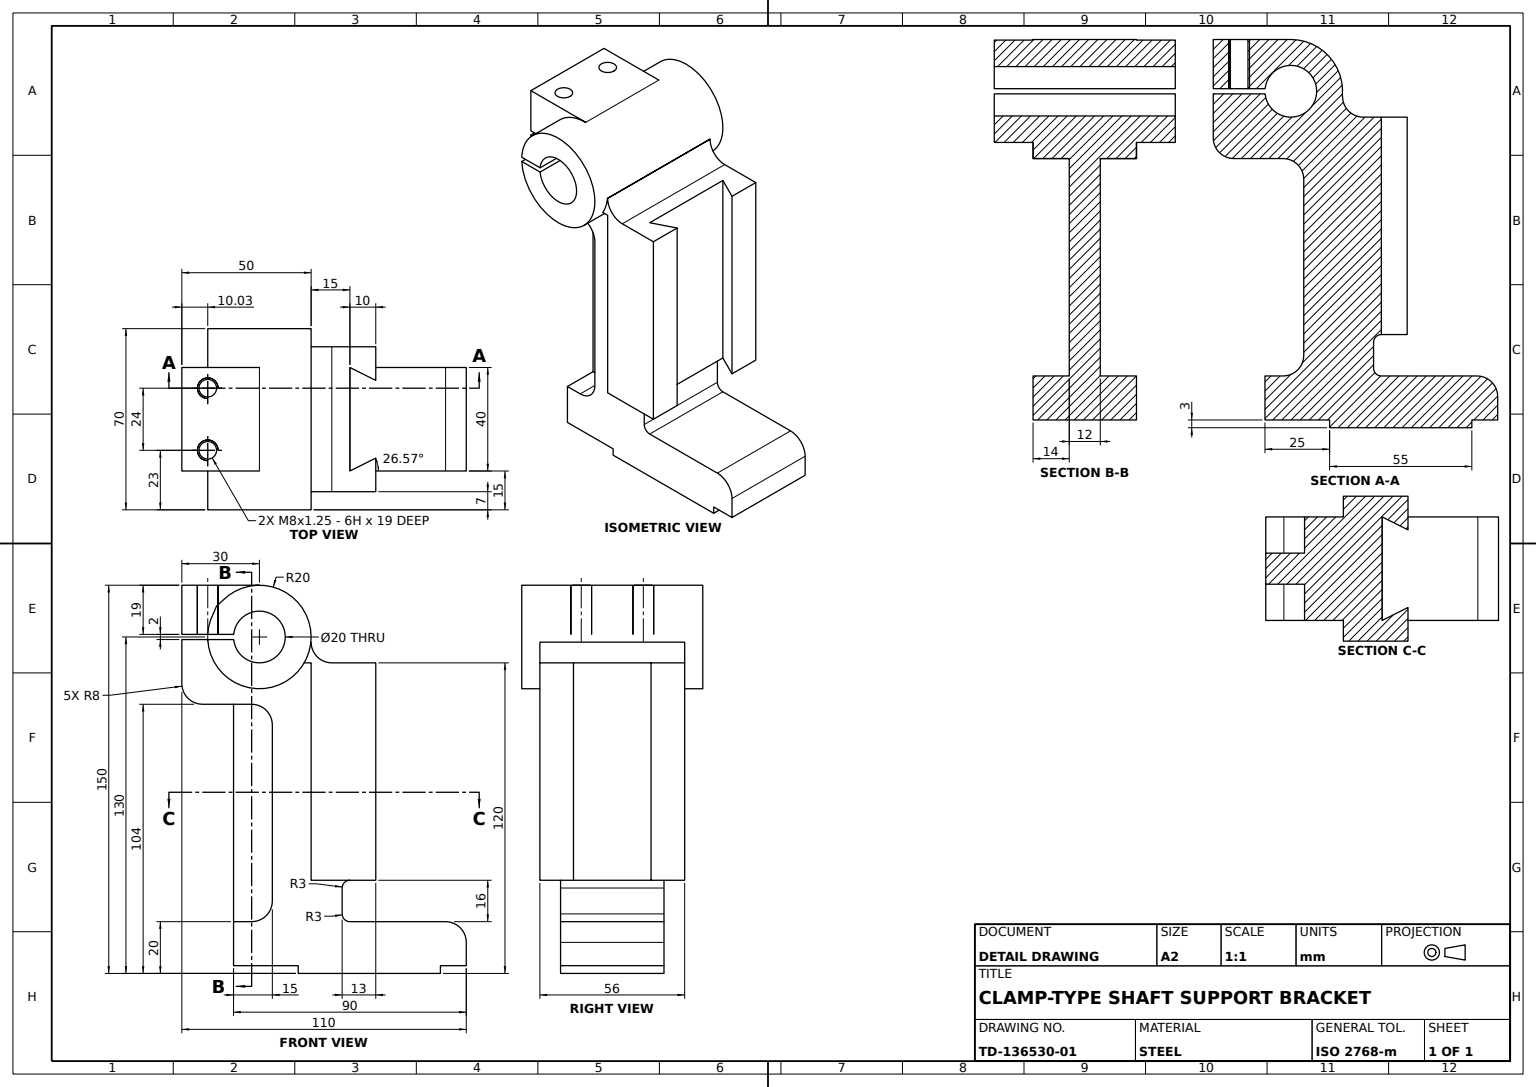
solid
v1 (28,120,-55)
v2 (15,120,-55)
e1 v1 v2 LINE
v3 (20,120,-45)
e2 v3 v2 LINE
v4 (-20,120,-45)
e3 v4 v3 LINE
v5 (-15,120,-55)
e4 v5 v4 LINE
v6 (-28,120,-55)
e5 v5 v6 LINE
v7 (-28,120,-38)
e6 v7 v6 LINE
v8 (28,120,-38)
e7 v8 v7 LINE
e8 v8 v1 LINE
face PLANE(AX(P(20,120,0),D(0,-1,0),D(0,0,-1))) rev [e1 -e2 -e3 -e4 e5 -e6 -e7 e8]
v9 (-20,0,-80)
v10 (20,0,-80)
e9 v9 v10 LINE
v11 (-20,3,-80)
e10 v11 v9 LINE
v12 (20,3,-80)
e11 v11 v12 LINE
e12 v12 v10 LINE
face PLANE(AX(P(-35.001,0,-80),D(0,0,1),D(1,0,0))) rev [-e9 -e10 e11 e12]
v13 (-20,36,-45)
e13 v13 v4 LINE
v14 (20,36,-45)
e14 v14 v3 LINE
e15 v14 v13 LINE
face PLANE(AX(P(-20,-0.001,-45),D(0,0,1),D(1,0,0))) rev [e13 e3 -e14 e15]
v15 (-28,120,-30)
v16 (-20,120,-30)
e16 v15 v16 LINE
v17 (-20,120,-27.320508)
e17 v16 v17 LINE
v18 (-28,120,-27.320508)
e18 v17 v18 LINE
e19 v18 v15 LINE
face PLANE(AX(P(-28,120,-23),D(0,1,0),D(0,0,1))) rev [e16 e17 e18 e19]
v19 (-28,128,-30)
e20 v19 v7 CIRCLE(AX(P(-28,128,-38),D(1,0,0),D(0,0,-1)),8)
v20 (28,128,-30)
e21 v20 v19 LINE
e22 v20 v8 CIRCLE(AX(P(28,128,-38),D(1,0,0),D(0,0,-1)),8)
face CYL(AX(P(28,128,-38),D(-1,0,0),D(0,0,1)),8) rev [-e20 -e21 e22 e7]
v21 (-20,112,20)
v22 (20,112,20)
e23 v21 v22 LINE
v23 (-20,104,12)
e24 v23 v21 CIRCLE(AX(P(-20,112,12),D(-1,0,0),D(0,0,1)),8)
v24 (20,104,12)
e25 v24 v23 LINE
e26 v22 v24 CIRCLE(AX(P(20,112,12),D(1,0,0),D(0,0,1)),8)
face CYL(AX(P(-20,112,12),D(-1,0,0),D(0,0,1)),8) [-e23 -e24 -e25 -e26]
v25 (20,150,20)
v26 (20,150,-10)
e27 v25 v26 LINE
v27 (20,131,20)
e28 v27 v25 LINE
v28 (20,131,9.974984)
e29 v27 v28 LINE
e30 v26 v28 CIRCLE(AX(P(20,130,-10),D(1,0,0),D(0,0,1)),20)
face PLANE(AX(P(20,33,-45),D(-1,0,0),D(0,0,1))) rev [-e27 -e28 e29 -e30]
v29 (6,20,-7)
v30 (6,28,-15)
e31 v29 v30 CIRCLE(AX(P(6,28,-7),D(1,0,0),D(0,0,1)),8)
v31 (6,96,-15)
e32 v30 v31 LINE
v32 (6,104,-7)
e33 v31 v32 CIRCLE(AX(P(6,96,-7),D(1,0,0),D(0,0,1)),8)
v33 (6,104,0)
e34 v32 v33 LINE
v34 (6,20,0)
e35 v33 v34 LINE
e36 v34 v29 LINE
face PLANE(AX(P(6,0,0),D(-1,0,0),D(0,0,1))) rev [e31 e32 e33 e34 e35 e36]
v35 (20,12,-90)
v36 (20,20,-82)
e37 v35 v36 CIRCLE(AX(P(20,12,-82),D(1,0,0),D(0,0,1)),8)
v37 (-20,12,-90)
e38 v37 v35 LINE
v38 (-20,20,-82)
e39 v38 v37 CIRCLE(AX(P(-20,12,-82),D(-1,0,0),D(0,0,1)),8)
e40 v36 v38 LINE
face CYL(AX(P(20,12,-82),D(-1,0,0),D(0,0,1)),8) [-e37 -e38 -e39 -e40]
v39 (-20,0,-25)
v40 (20,0,-25)
e41 v39 v40 LINE
e42 v39 v9 LINE
e43 v40 v10 LINE
face PLANE(AX(P(20,0,0),D(0,1,0),D(0,0,1))) rev [-e41 e42 e9 -e43]
v41 (12,131,13.374984)
v42 (12,131,6.574984)
e44 v41 v42 CIRCLE(AX(P(12,131,9.974984),D(0,1,0),D(0,0,1)),3.4)
v43 (12,150,13.374984)
e45 v41 v43 LINE
v44 (12,150,6.574984)
e46 v43 v44 CIRCLE(AX(P(12,150,9.974984),D(0,1,0),D(0,0,1)),3.4)
e47 v42 v44 LINE
face CYL(AX(P(12,150,9.974984),D(0,1,0),D(0,0,1)),3.4) rev [-e44 e45 e46 -e47]
v45 (-12,131,6.574984)
v46 (-12,131,13.374984)
e48 v45 v46 CIRCLE(AX(P(-12,131,9.974984),D(0,1,0),D(0,0,1)),3.4)
v47 (-12,150,6.574984)
e49 v45 v47 LINE
v48 (-12,150,13.374984)
e50 v47 v48 CIRCLE(AX(P(-12,150,9.974984),D(0,1,0),D(0,0,1)),3.4)
e51 v46 v48 LINE
face CYL(AX(P(-12,150,9.974984),D(0,1,0),D(0,0,1)),3.4) rev [-e48 e49 e50 -e51]
v49 (-20,3,-25)
v50 (-20,3,0)
e52 v49 v50 LINE
v51 (20,3,-25)
e53 v49 v51 LINE
v52 (20,3,0)
e54 v51 v52 LINE
e55 v50 v52 LINE
face PLANE(AX(P(-35.001,3,0),D(0,1,0),D(0,0,1))) rev [-e52 e53 e54 -e55]
v53 (20,20,-45)
e56 v36 v53 LINE
v54 (-20,20,-45)
e57 v38 v54 LINE
e58 v53 v54 LINE
face PLANE(AX(P(20,20,-90),D(0,-1,0),D(0,0,-1))) rev [-e56 e40 e57 -e58]
v55 (20,20,0)
e59 v55 v52 LINE
e60 v34 v55 LINE
v56 (-6,104,0)
e61 v56 v33 LINE
v57 (-6,20,0)
e62 v57 v56 LINE
v58 (-20,20,0)
e63 v57 v58 LINE
e64 v58 v50 LINE
face PLANE(AX(P(20,0,0),D(0,0,-1),D(-1,0,0))) rev [e55 -e59 -e60 -e35 -e61 -e62 e63 e64]
e65 v39 v49 LINE
e66 v40 v51 LINE
face PLANE(AX(P(-35.001,0,-25),D(0,0,-1),D(-1,0,0))) rev [-e65 e41 e66 -e53]
v59 (-28,128,-29.899749)
e67 v18 v59 CIRCLE(AX(P(-28,130,-10),D(1,0,0),D(0,0,-1)),20)
e68 v59 v19 LINE
v60 (-28,36,-55)
e69 v6 v60 LINE
v61 (-28,36,-30)
e70 v61 v60 LINE
e71 v15 v61 LINE
face PLANE(AX(P(-28,0,0),D(1,0,0),D(0,0,-1))) rev [-e19 e67 e68 e20 e6 e69 -e70 -e71]
v62 (-35,131,-0.050126)
v63 (35,131,-0.050126)
e72 v62 v63 LINE
v64 (-35,129,-0.050126)
e73 v64 v62 CIRCLE(AX(P(-35,130,-10),D(1,0,0),D(0,0,-1)),10)
v65 (35,129,-0.050126)
e74 v64 v65 LINE
e75 v65 v63 CIRCLE(AX(P(35,130,-10),D(1,0,0),D(0,0,-1)),10)
face CYL(AX(P(35,130,-10),D(-1,0,0),D(0,0,1)),10) rev [-e72 -e73 e74 e75]
v66 (20,28,-15)
e76 v30 v66 LINE
v67 (20,96,-15)
e77 v66 v67 LINE
e78 v67 v31 LINE
face PLANE(AX(P(6,104,-15),D(0,0,-1),D(0,1,0))) rev [e76 e77 e78 -e32]
e79 v48 v47 CIRCLE(AX(P(-12,150,9.974984),D(0,1,0),D(0,0,1)),3.4)
e80 v46 v45 CIRCLE(AX(P(-12,131,9.974984),D(0,1,0),D(0,0,1)),3.4)
face CYL(AX(P(-12,150,9.974984),D(0,1,0),D(0,0,1)),3.4) rev [e51 e79 -e49 -e80]
v68 (-20,150,-10)
v69 (-20,131,9.974984)
e81 v68 v69 CIRCLE(AX(P(-20,130,-10),D(1,0,0),D(0,0,1)),20)
v70 (-20,131,20)
e82 v70 v69 LINE
v71 (-20,150,20)
e83 v70 v71 LINE
e84 v68 v71 LINE
face PLANE(AX(P(-20,33,-45),D(-1,0,0),D(0,0,1))) [e81 -e82 e83 -e84]
v72 (20,129,20)
e85 v22 v72 LINE
v73 (-20,129,20)
e86 v73 v72 LINE
e87 v21 v73 LINE
face PLANE(AX(P(-20,104,20),D(0,0,1),D(1,0,0))) [e23 e85 -e86 -e87]
v74 (28,36,-30)
v75 (28,36,-55)
e88 v74 v75 LINE
v76 (20,36,-30)
e89 v74 v76 LINE
e90 v76 v14 LINE
v77 (15,36,-55)
e91 v77 v14 LINE
e92 v75 v77 LINE
face PLANE(AX(P(20,36,-45),D(0,1,0),D(0,0,1))) rev [-e88 e89 e90 -e91 -e92]
e93 v77 v2 LINE
face PLANE(AX(P(20,-0.001,-45),D(0.894427191,0,-0.447213595),D(-0.447213595,0,-0.894427191))) rev [e91 e14 e2 -e93]
v78 (20,23,-42)
v79 (-20,23,-42)
e94 v78 v79 LINE
e95 v53 v78 CIRCLE(AX(P(20,23,-45),D(-1,0,0),D(0,0,1)),3)
e96 v54 v79 CIRCLE(AX(P(-20,23,-45),D(-1,0,0),D(0,0,1)),3)
face CYL(AX(P(20,23,-45),D(-1,0,0),D(0,0,1)),3) rev [-e94 -e95 e58 e96]
v80 (20,120,-30)
v81 (28,120,-30)
e97 v80 v81 LINE
e98 v80 v76 LINE
e99 v81 v74 LINE
face PLANE(AX(P(28,0,-30),D(0,0,-1),D(0,1,0))) rev [-e97 e98 -e89 -e99]
v82 (-20,20,-7)
e100 v82 v58 LINE
v83 (-20,28,-15)
e101 v82 v83 CIRCLE(AX(P(-20,28,-7),D(1,0,0),D(0,0,1)),8)
v84 (-20,96,-15)
e102 v84 v83 LINE
v85 (-20,104,-7)
e103 v84 v85 CIRCLE(AX(P(-20,96,-7),D(1,0,0),D(0,0,1)),8)
e104 v85 v23 LINE
v86 (-20,129,9.974984)
e105 v73 v86 LINE
e106 v86 v17 CIRCLE(AX(P(-20,130,-10),D(1,0,0),D(0,0,1)),20)
v87 (-20,36,-30)
e107 v16 v87 LINE
e108 v87 v13 LINE
v88 (-20,33,-42)
e109 v88 v13 CIRCLE(AX(P(-20,33,-45),D(-1,0,0),D(0,0,1)),3)
e110 v79 v88 LINE
v89 (-20,3,-90)
e111 v89 v37 LINE
e112 v89 v11 LINE
face PLANE(AX(P(-20,33,-45),D(-1,0,0),D(0,0,1))) [-e42 e65 e52 -e64 -e100 e101 -e102 e103 e104 e24 e87 e105 e106 -e17 e107 e108 -e109 -e110 -e96 -e57 e39 -e111 e112 e10]
e113 v26 v68 LINE
e114 v71 v25 LINE
e115 v44 v43 CIRCLE(AX(P(12,150,9.974984),D(0,1,0),D(0,0,1)),3.4)
face PLANE(AX(P(0,150,0),D(0,1,0),D(0,0,1))) [e27 e113 e84 e114] [-e79 -e50] [-e46 -e115]
v90 (20,129,9.974984)
v91 (35,129,9.974984)
e116 v90 v91 LINE
v92 (20,120,-27.320508)
e117 v90 v92 CIRCLE(AX(P(20,130,-10),D(1,0,0),D(0,0,1)),20)
v93 (28,120,-27.320508)
e118 v93 v92 LINE
v94 (28,128,-29.899749)
e119 v94 v93 CIRCLE(AX(P(28,130,-10),D(-1,0,0),D(0,0,1)),20)
e120 v59 v94 LINE
v95 (-35,129,9.974984)
e121 v95 v86 LINE
v96 (-35,131,9.974984)
e122 v95 v96 CIRCLE(AX(P(-35,130,-10),D(1,0,0),D(0,0,-1)),20)
e123 v96 v69 LINE
v97 (35,131,9.974984)
e124 v28 v97 LINE
e125 v91 v97 CIRCLE(AX(P(35,130,-10),D(1,0,0),D(0,0,-1)),20)
face CYL(AX(P(35,130,-10),D(-1,0,0),D(0,0,1)),20) [-e116 e117 -e118 -e119 -e120 -e67 -e18 -e106 -e121 e122 e123 -e81 -e113 e30 e124 -e125]
e126 v93 v81 LINE
e127 v80 v92 LINE
face PLANE(AX(P(-28,120,-23),D(0,1,0),D(0,0,1))) rev [-e126 e118 -e127 e97]
v98 (20,3,-90)
e128 v98 v35 LINE
e129 v89 v98 LINE
face PLANE(AX(P(20,0,-90),D(0,0,1),D(1,0,0))) rev [e38 -e128 -e129 e111]
e130 v1 v75 LINE
face PLANE(AX(P(20,36,-55),D(0,0,1),D(0,-1,0))) rev [e93 -e1 e130 e92]
e131 v87 v61 LINE
v99 (-15,36,-55)
e132 v99 v60 LINE
e133 v13 v99 LINE
face PLANE(AX(P(20,36,-45),D(0,1,0),D(0,0,1))) rev [-e108 e131 e70 -e132 -e133]
e134 v99 v5 LINE
face PLANE(AX(P(-15,-0.001,-55),D(-0.894427191,0,-0.447213595),D(-0.447213595,0,0.894427191))) rev [e134 e4 -e13 e133]
e135 v70 v27 LINE
face PLANE(AX(P(-20,104,20),D(0,0,1),D(1,0,0))) [-e83 e135 e28 -e114]
e136 v94 v20 LINE
face PLANE(AX(P(28,0,0),D(1,0,0),D(0,0,-1))) [e99 e88 -e130 -e8 -e22 -e136 e119 e126]
face PLANE(AX(P(28,0,-30),D(0,0,-1),D(0,1,0))) rev [-e107 -e16 e71 -e131]
v100 (20,33,-42)
e137 v100 v88 LINE
e138 v100 v14 CIRCLE(AX(P(20,33,-45),D(-1,0,0),D(0,0,1)),3)
face CYL(AX(P(20,33,-45),D(-1,0,0),D(0,0,1)),3) rev [e137 e109 -e15 -e138]
e139 v97 v63 LINE
e140 v91 v65 LINE
face PLANE(AX(P(35,130,-10),D(1,0,0),D(0,0,-1))) [e139 -e75 -e140 e125]
v101 (-6,96,-15)
e141 v101 v84 LINE
v102 (-6,28,-15)
e142 v83 v102 LINE
e143 v101 v102 LINE
face PLANE(AX(P(-6,33,-15),D(0,0,-1),D(0,1,0))) rev [e141 e102 e142 -e143]
e144 v98 v12 LINE
face PLANE(AX(P(-35.001,3,-90),D(0,1,0),D(0,0,1))) rev [e129 e144 -e11 -e112]
e145 v78 v100 LINE
e146 v72 v90 LINE
v103 (20,104,-7)
e147 v24 v103 LINE
e148 v103 v67 CIRCLE(AX(P(20,96,-7),D(-1,0,0),D(0,0,1)),8)
v104 (20,20,-7)
e149 v66 v104 CIRCLE(AX(P(20,28,-7),D(-1,0,0),D(0,0,1)),8)
e150 v55 v104 LINE
face PLANE(AX(P(20,33,-45),D(-1,0,0),D(0,0,1))) rev [e128 e37 e56 e95 e145 e138 -e90 -e98 e127 -e117 -e146 -e85 e26 e147 e148 -e77 e149 -e150 e59 -e54 -e66 e43 -e12 -e144]
face PLANE(AX(P(20,36,-55),D(0,0,1),D(0,-1,0))) rev [-e134 e132 -e69 -e5]
v105 (-6,20,-7)
e151 v105 v57 LINE
e152 v105 v82 LINE
face PLANE(AX(P(-6,20,-45),D(0,-1,0),D(0,0,-1))) rev [-e151 e152 e100 -e63]
e153 v64 v95 LINE
face PLANE(AX(P(0,129,0),D(0,1,0),D(0,0,1))) [-e105 e86 e146 e116 e140 -e74 e153 e121]
face PLANE(AX(P(20,23,-42),D(0,0,1),D(1,0,0))) rev [e94 e110 -e137 -e145]
e154 v32 v103 LINE
face CYL(AX(P(0,96,-7),D(-1,0,0),D(0,0,1)),8) rev [-e33 -e78 -e148 -e154]
e155 v62 v96 LINE
e156 v42 v41 CIRCLE(AX(P(12,131,9.974984),D(0,1,0),D(0,0,1)),3.4)
face PLANE(AX(P(0,131,0),D(0,1,0),D(0,0,1))) rev [-e29 -e135 e82 -e123 -e155 e72 -e139 -e124] [e80 e48] [e156 e44]
v106 (-6,104,-7)
e157 v85 v106 LINE
e158 v56 v106 LINE
face PLANE(AX(P(0,104,0),D(0,1,0),D(0,0,1))) rev [e157 -e158 e61 -e34 e154 -e147 e25 -e104]
e159 v102 v105 CIRCLE(AX(P(-6,28,-7),D(-1,0,0),D(0,0,1)),8)
face CYL(AX(P(-6,28,-7),D(1,0,0),D(0,0,-1)),8) rev [-e101 -e152 -e159 -e142]
e160 v106 v101 CIRCLE(AX(P(-6,96,-7),D(-1,0,0),D(0,0,1)),8)
face CYL(AX(P(-6,96,-7),D(1,0,0),D(0,0,-1)),8) rev [-e157 -e103 -e141 -e160]
face PLANE(AX(P(-35,130,-10),D(1,0,0),D(0,0,-1))) rev [e73 e155 -e122 -e153]
face CYL(AX(P(12,150,9.974984),D(0,1,0),D(0,0,1)),3.4) rev [e47 e115 -e45 -e156]
e161 v104 v29 LINE
face CYL(AX(P(6,28,-7),D(-1,0,0),D(0,0,1)),8) rev [-e31 -e161 -e149 -e76]
face PLANE(AX(P(28,128,-23),D(0,-1,0),D(0,0,-1))) rev [e21 -e68 e120 e136]
face PLANE(AX(P(6,20,-15),D(0,-1,0),D(0,0,-1))) rev [e150 e161 -e36 e60]
face PLANE(AX(P(-6,0,0),D(-1,0,0),D(0,0,1))) [e160 e143 e159 e151 e62 e158]
